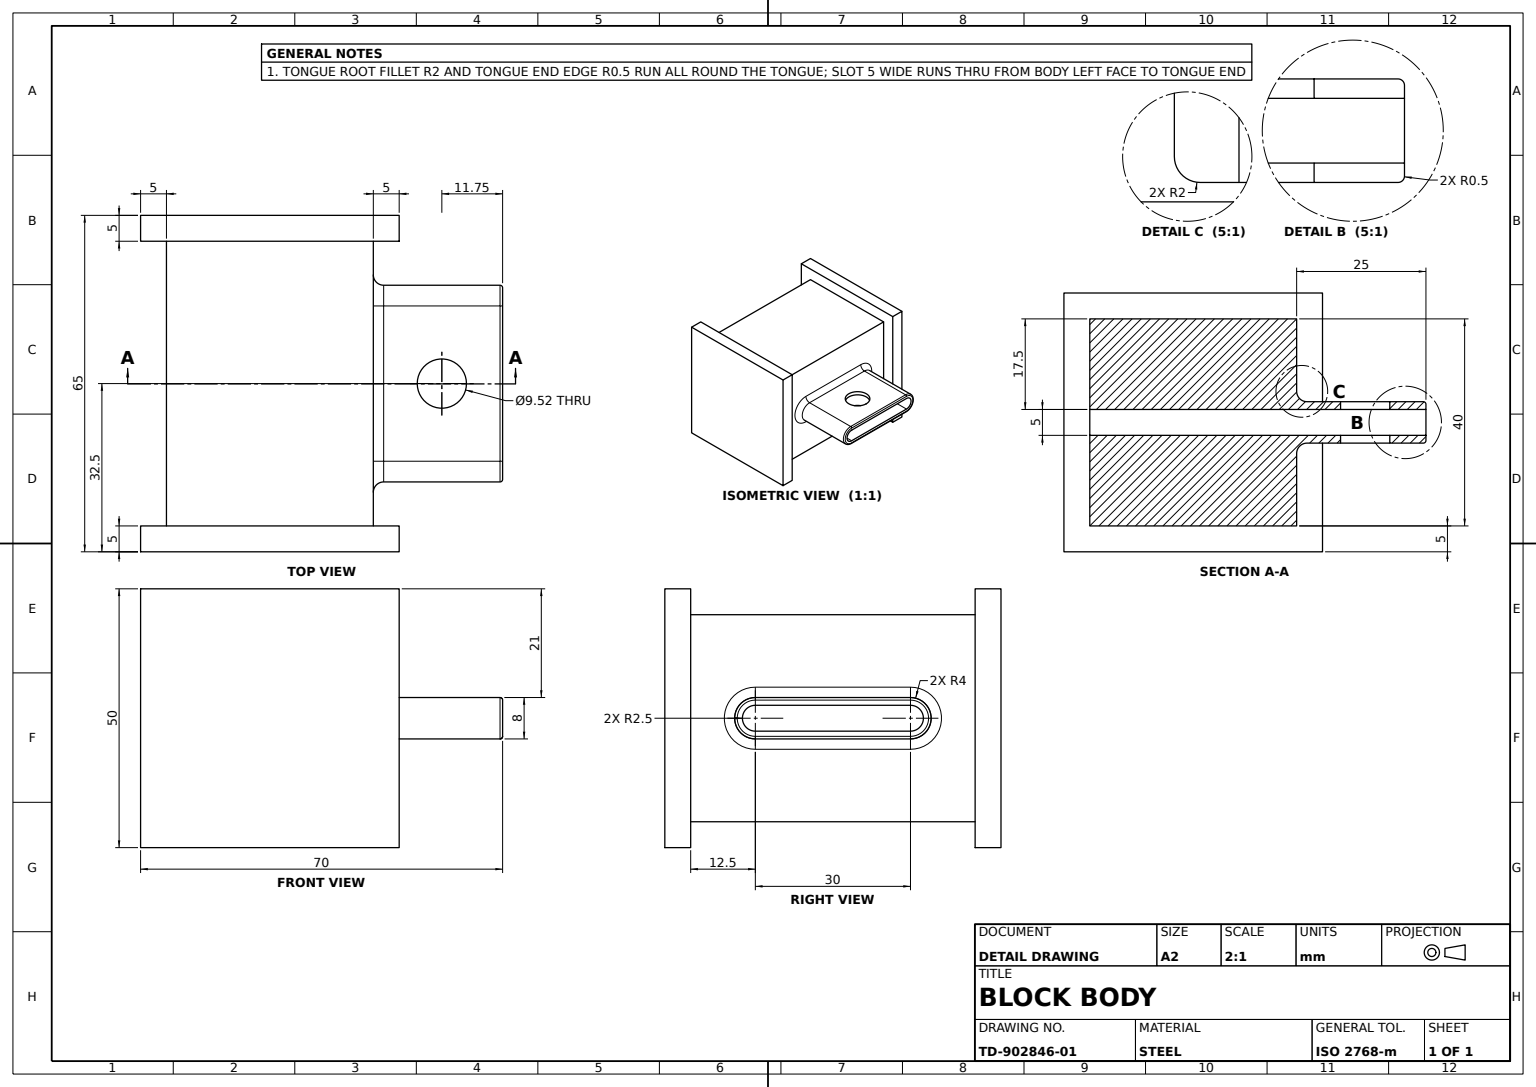
ISO-10303-21;
HEADER;
FILE_DESCRIPTION((''),'2;1');
FILE_NAME('','',(''),(''),'','','');
FILE_SCHEMA(('AUTOMOTIVE_DESIGN'));
ENDSEC;
DATA;
#1=APPLICATION_CONTEXT('');
#2=PRODUCT_CONTEXT('',#1,'mechanical');
#3=PRODUCT('','','',(#2));
#4=PRODUCT_DEFINITION_FORMATION('','',#3);
#5=PRODUCT_DEFINITION_CONTEXT('',#1,'design');
#6=PRODUCT_DEFINITION('','',#4,#5);
#7=PRODUCT_DEFINITION_SHAPE('','',#6);
#8=(LENGTH_UNIT()NAMED_UNIT(*)SI_UNIT(.MILLI.,.METRE.));
#9=(NAMED_UNIT(*)PLANE_ANGLE_UNIT()SI_UNIT($,.RADIAN.));
#10=(NAMED_UNIT(*)SI_UNIT($,.STERADIAN.)SOLID_ANGLE_UNIT());
#11=UNCERTAINTY_MEASURE_WITH_UNIT(LENGTH_MEASURE(1.E-05),#8,'distance_accuracy_value','');
#12=(GEOMETRIC_REPRESENTATION_CONTEXT(3)GLOBAL_UNCERTAINTY_ASSIGNED_CONTEXT((#11))GLOBAL_UNIT_ASSIGNED_CONTEXT((#8,#9,#10))REPRESENTATION_CONTEXT('',''));
#13=CARTESIAN_POINT('',(50.,0.,0.));
#14=VERTEX_POINT('',#13);
#15=CARTESIAN_POINT('',(50.,50.,0.));
#16=VERTEX_POINT('',#15);
#17=DIRECTION('',(0.,1.,0.));
#18=VECTOR('',#17,1000.);
#19=LINE('',#15,#18);
#20=EDGE_CURVE('',#14,#16,#19,.T.);
#21=ORIENTED_EDGE('',*,*,#20,.F.);
#22=CARTESIAN_POINT('',(0.,0.,0.));
#23=VERTEX_POINT('',#22);
#24=DIRECTION('',(1.,0.,0.));
#25=VECTOR('',#24,1000.);
#26=LINE('',#13,#25);
#27=EDGE_CURVE('',#23,#14,#26,.T.);
#28=ORIENTED_EDGE('',*,*,#27,.F.);
#29=CARTESIAN_POINT('',(0.,50.,0.));
#30=VERTEX_POINT('',#29);
#31=DIRECTION('',(0.,-1.,0.));
#32=VECTOR('',#31,1000.);
#33=LINE('',#22,#32);
#34=EDGE_CURVE('',#30,#23,#33,.T.);
#35=ORIENTED_EDGE('',*,*,#34,.F.);
#36=DIRECTION('',(-1.,0.,0.));
#37=VECTOR('',#36,1000.);
#38=LINE('',#29,#37);
#39=EDGE_CURVE('',#16,#30,#38,.T.);
#40=ORIENTED_EDGE('',*,*,#39,.F.);
#41=EDGE_LOOP('',(#21,#28,#35,#40));
#42=FACE_OUTER_BOUND('',#41,.T.);
#43=DIRECTION('',(0.,0.,-1.));
#44=AXIS2_PLACEMENT_3D('',#22,#43,#36);
#45=PLANE('',#44);
#46=ADVANCED_FACE('',(#42),#45,.T.);
#47=CARTESIAN_POINT('',(63.00949,29.,32.5));
#48=VERTEX_POINT('',#47);
#49=CARTESIAN_POINT('',(63.00949,27.5,32.5));
#50=VERTEX_POINT('',#49);
#51=CARTESIAN_POINT('',(63.00949,50.,32.5));
#52=LINE('',#51,#32);
#53=EDGE_CURVE('',#48,#50,#52,.T.);
#54=ORIENTED_EDGE('',*,*,#53,.F.);
#55=CARTESIAN_POINT('',(53.49051,29.,32.5));
#56=VERTEX_POINT('',#55);
#57=CARTESIAN_POINT('',(58.25,29.,32.5));
#58=AXIS2_PLACEMENT_3D('',#57,#17,#36);
#59=CIRCLE('',#58,4.75949);
#60=EDGE_CURVE('',#48,#56,#59,.T.);
#61=ORIENTED_EDGE('',*,*,#60,.T.);
#62=CARTESIAN_POINT('',(53.49051,27.5,32.5));
#63=VERTEX_POINT('',#62);
#64=CARTESIAN_POINT('',(53.49051,50.,32.5));
#65=LINE('',#64,#32);
#66=EDGE_CURVE('',#56,#63,#65,.T.);
#67=ORIENTED_EDGE('',*,*,#66,.T.);
#68=CARTESIAN_POINT('',(58.25,27.5,32.5));
#69=AXIS2_PLACEMENT_3D('',#68,#17,#36);
#70=CIRCLE('',#69,4.75949);
#71=EDGE_CURVE('',#50,#63,#70,.T.);
#72=ORIENTED_EDGE('',*,*,#71,.F.);
#73=EDGE_LOOP('',(#54,#61,#67,#72));
#74=FACE_OUTER_BOUND('',#73,.T.);
#75=CARTESIAN_POINT('',(58.25,50.,32.5));
#76=AXIS2_PLACEMENT_3D('',#75,#31,#24);
#77=CYLINDRICAL_SURFACE('',#76,4.75949);
#78=ADVANCED_FACE('',(#74),#77,.F.);
#79=CARTESIAN_POINT('',(5.,22.5,47.5));
#80=VERTEX_POINT('',#79);
#81=CARTESIAN_POINT('',(5.,22.5,17.5));
#82=VERTEX_POINT('',#81);
#83=CARTESIAN_POINT('',(5.,22.5,60.));
#84=VECTOR('',#43,1000.);
#85=LINE('',#83,#84);
#86=EDGE_CURVE('',#80,#82,#85,.T.);
#87=ORIENTED_EDGE('',*,*,#86,.T.);
#88=CARTESIAN_POINT('',(5.,27.5,17.5));
#89=VERTEX_POINT('',#88);
#90=CARTESIAN_POINT('',(5.,25.,17.5));
#91=AXIS2_PLACEMENT_3D('',#90,#24,#17);
#92=CIRCLE('',#91,2.5);
#93=EDGE_CURVE('',#82,#89,#92,.T.);
#94=ORIENTED_EDGE('',*,*,#93,.T.);
#95=CARTESIAN_POINT('',(5.,27.5,47.5));
#96=VERTEX_POINT('',#95);
#97=CARTESIAN_POINT('',(5.,27.5,60.));
#98=DIRECTION('',(0.,0.,1.));
#99=VECTOR('',#98,1000.);
#100=LINE('',#97,#99);
#101=EDGE_CURVE('',#89,#96,#100,.T.);
#102=ORIENTED_EDGE('',*,*,#101,.T.);
#103=CARTESIAN_POINT('',(5.,25.,47.5));
#104=AXIS2_PLACEMENT_3D('',#103,#24,#17);
#105=CIRCLE('',#104,2.5);
#106=EDGE_CURVE('',#96,#80,#105,.T.);
#107=ORIENTED_EDGE('',*,*,#106,.T.);
#108=EDGE_LOOP('',(#87,#94,#102,#107));
#109=FACE_BOUND('',#108,.T.);
#110=CARTESIAN_POINT('',(5.,45.,60.));
#111=VERTEX_POINT('',#110);
#112=CARTESIAN_POINT('',(5.,45.,5.));
#113=VERTEX_POINT('',#112);
#114=LINE('',#110,#84);
#115=EDGE_CURVE('',#111,#113,#114,.T.);
#116=ORIENTED_EDGE('',*,*,#115,.T.);
#117=CARTESIAN_POINT('',(5.,5.,5.));
#118=VERTEX_POINT('',#117);
#119=LINE('',#112,#32);
#120=EDGE_CURVE('',#113,#118,#119,.T.);
#121=ORIENTED_EDGE('',*,*,#120,.T.);
#122=CARTESIAN_POINT('',(5.,5.,60.));
#123=VERTEX_POINT('',#122);
#124=LINE('',#122,#84);
#125=EDGE_CURVE('',#123,#118,#124,.T.);
#126=ORIENTED_EDGE('',*,*,#125,.F.);
#127=LINE('',#110,#32);
#128=EDGE_CURVE('',#111,#123,#127,.T.);
#129=ORIENTED_EDGE('',*,*,#128,.F.);
#130=EDGE_LOOP('',(#116,#121,#126,#129));
#131=FACE_OUTER_BOUND('',#130,.T.);
#132=AXIS2_PLACEMENT_3D('',#110,#24,#17);
#133=PLANE('',#132);
#134=ADVANCED_FACE('',(#109,#131),#133,.F.);
#135=CARTESIAN_POINT('',(45.,5.,5.));
#136=VERTEX_POINT('',#135);
#137=LINE('',#117,#25);
#138=EDGE_CURVE('',#118,#136,#137,.T.);
#139=ORIENTED_EDGE('',*,*,#138,.T.);
#140=CARTESIAN_POINT('',(45.,5.,60.));
#141=VERTEX_POINT('',#140);
#142=LINE('',#140,#84);
#143=EDGE_CURVE('',#141,#136,#142,.T.);
#144=ORIENTED_EDGE('',*,*,#143,.F.);
#145=LINE('',#122,#25);
#146=EDGE_CURVE('',#123,#141,#145,.T.);
#147=ORIENTED_EDGE('',*,*,#146,.F.);
#148=ORIENTED_EDGE('',*,*,#125,.T.);
#149=EDGE_LOOP('',(#139,#144,#147,#148));
#150=FACE_OUTER_BOUND('',#149,.T.);
#151=AXIS2_PLACEMENT_3D('',#122,#17,#98);
#152=PLANE('',#151);
#153=ADVANCED_FACE('',(#150),#152,.F.);
#154=CARTESIAN_POINT('',(50.,50.,60.));
#155=VERTEX_POINT('',#154);
#156=CARTESIAN_POINT('',(0.,50.,60.));
#157=VERTEX_POINT('',#156);
#158=LINE('',#156,#37);
#159=EDGE_CURVE('',#155,#157,#158,.T.);
#160=ORIENTED_EDGE('',*,*,#159,.T.);
#161=CARTESIAN_POINT('',(0.,50.,65.));
#162=VERTEX_POINT('',#161);
#163=LINE('',#161,#84);
#164=EDGE_CURVE('',#162,#157,#163,.T.);
#165=ORIENTED_EDGE('',*,*,#164,.F.);
#166=CARTESIAN_POINT('',(50.,50.,65.));
#167=VERTEX_POINT('',#166);
#168=LINE('',#161,#37);
#169=EDGE_CURVE('',#167,#162,#168,.T.);
#170=ORIENTED_EDGE('',*,*,#169,.F.);
#171=LINE('',#166,#84);
#172=EDGE_CURVE('',#167,#155,#171,.T.);
#173=ORIENTED_EDGE('',*,*,#172,.T.);
#174=EDGE_LOOP('',(#160,#165,#170,#173));
#175=FACE_OUTER_BOUND('',#174,.T.);
#176=AXIS2_PLACEMENT_3D('',#161,#31,#43);
#177=PLANE('',#176);
#178=ADVANCED_FACE('',(#175),#177,.F.);
#179=CARTESIAN_POINT('',(47.,29.,17.5));
#180=VERTEX_POINT('',#179);
#181=CARTESIAN_POINT('',(47.,29.,47.5));
#182=VERTEX_POINT('',#181);
#183=LINE('',#181,#99);
#184=EDGE_CURVE('',#180,#182,#183,.T.);
#185=ORIENTED_EDGE('',*,*,#184,.F.);
#186=CARTESIAN_POINT('',(45.,31.,17.5));
#187=VERTEX_POINT('',#186);
#188=CARTESIAN_POINT('',(47.,31.,17.5));
#189=AXIS2_PLACEMENT_3D('',#188,#43,#36);
#190=CIRCLE('',#189,2.);
#191=EDGE_CURVE('',#180,#187,#190,.T.);
#192=ORIENTED_EDGE('',*,*,#191,.T.);
#193=CARTESIAN_POINT('',(45.,31.,47.5));
#194=VERTEX_POINT('',#193);
#195=CARTESIAN_POINT('',(45.,31.,60.));
#196=LINE('',#195,#84);
#197=EDGE_CURVE('',#194,#187,#196,.T.);
#198=ORIENTED_EDGE('',*,*,#197,.F.);
#199=CARTESIAN_POINT('',(47.,31.,47.5));
#200=AXIS2_PLACEMENT_3D('',#199,#43,#36);
#201=CIRCLE('',#200,2.);
#202=EDGE_CURVE('',#182,#194,#201,.T.);
#203=ORIENTED_EDGE('',*,*,#202,.F.);
#204=EDGE_LOOP('',(#185,#192,#198,#203));
#205=FACE_OUTER_BOUND('',#204,.T.);
#206=CARTESIAN_POINT('',(47.,31.,60.));
#207=AXIS2_PLACEMENT_3D('',#206,#43,#36);
#208=CYLINDRICAL_SURFACE('',#207,2.);
#209=ADVANCED_FACE('',(#205),#208,.F.);
#210=ORIENTED_EDGE('',*,*,#159,.F.);
#211=CARTESIAN_POINT('',(50.,0.,60.));
#212=VERTEX_POINT('',#211);
#213=LINE('',#154,#18);
#214=EDGE_CURVE('',#212,#155,#213,.T.);
#215=ORIENTED_EDGE('',*,*,#214,.F.);
#216=CARTESIAN_POINT('',(0.,0.,60.));
#217=VERTEX_POINT('',#216);
#218=LINE('',#211,#25);
#219=EDGE_CURVE('',#217,#212,#218,.T.);
#220=ORIENTED_EDGE('',*,*,#219,.F.);
#221=LINE('',#216,#32);
#222=EDGE_CURVE('',#157,#217,#221,.T.);
#223=ORIENTED_EDGE('',*,*,#222,.F.);
#224=EDGE_LOOP('',(#210,#215,#220,#223));
#225=FACE_OUTER_BOUND('',#224,.T.);
#226=ORIENTED_EDGE('',*,*,#128,.T.);
#227=ORIENTED_EDGE('',*,*,#146,.T.);
#228=CARTESIAN_POINT('',(45.,45.,60.));
#229=VERTEX_POINT('',#228);
#230=LINE('',#228,#18);
#231=EDGE_CURVE('',#141,#229,#230,.T.);
#232=ORIENTED_EDGE('',*,*,#231,.T.);
#233=LINE('',#110,#37);
#234=EDGE_CURVE('',#229,#111,#233,.T.);
#235=ORIENTED_EDGE('',*,*,#234,.T.);
#236=EDGE_LOOP('',(#226,#227,#232,#235));
#237=FACE_BOUND('',#236,.T.);
#238=AXIS2_PLACEMENT_3D('',#216,#43,#36);
#239=PLANE('',#238);
#240=ADVANCED_FACE('',(#225,#237),#239,.T.);
#241=CARTESIAN_POINT('',(45.,45.,5.));
#242=VERTEX_POINT('',#241);
#243=LINE('',#112,#37);
#244=EDGE_CURVE('',#242,#113,#243,.T.);
#245=ORIENTED_EDGE('',*,*,#244,.T.);
#246=ORIENTED_EDGE('',*,*,#115,.F.);
#247=ORIENTED_EDGE('',*,*,#234,.F.);
#248=LINE('',#228,#84);
#249=EDGE_CURVE('',#229,#242,#248,.T.);
#250=ORIENTED_EDGE('',*,*,#249,.T.);
#251=EDGE_LOOP('',(#245,#246,#247,#250));
#252=FACE_OUTER_BOUND('',#251,.T.);
#253=AXIS2_PLACEMENT_3D('',#110,#31,#43);
#254=PLANE('',#253);
#255=ADVANCED_FACE('',(#252),#254,.F.);
#256=CARTESIAN_POINT('',(69.5,21.,47.5));
#257=VERTEX_POINT('',#256);
#258=CARTESIAN_POINT('',(70.,21.5,47.5));
#259=VERTEX_POINT('',#258);
#260=CARTESIAN_POINT('',(69.5,21.5,47.5));
#261=AXIS2_PLACEMENT_3D('',#260,#98,#24);
#262=CIRCLE('',#261,0.5);
#263=EDGE_CURVE('',#257,#259,#262,.T.);
#264=ORIENTED_EDGE('',*,*,#263,.F.);
#265=CARTESIAN_POINT('',(69.5,21.,17.5));
#266=VERTEX_POINT('',#265);
#267=LINE('',#256,#99);
#268=EDGE_CURVE('',#266,#257,#267,.T.);
#269=ORIENTED_EDGE('',*,*,#268,.F.);
#270=CARTESIAN_POINT('',(70.,21.5,17.5));
#271=VERTEX_POINT('',#270);
#272=CARTESIAN_POINT('',(69.5,21.5,17.5));
#273=AXIS2_PLACEMENT_3D('',#272,#98,#24);
#274=CIRCLE('',#273,0.5);
#275=EDGE_CURVE('',#266,#271,#274,.T.);
#276=ORIENTED_EDGE('',*,*,#275,.T.);
#277=LINE('',#270,#84);
#278=EDGE_CURVE('',#259,#271,#277,.T.);
#279=ORIENTED_EDGE('',*,*,#278,.F.);
#280=EDGE_LOOP('',(#264,#269,#276,#279));
#281=FACE_OUTER_BOUND('',#280,.T.);
#282=CARTESIAN_POINT('',(69.5,21.5,0.));
#283=AXIS2_PLACEMENT_3D('',#282,#98,#24);
#284=CYLINDRICAL_SURFACE('',#283,0.5);
#285=ADVANCED_FACE('',(#281),#284,.T.);
#286=CARTESIAN_POINT('',(50.,0.,65.));
#287=VERTEX_POINT('',#286);
#288=LINE('',#166,#18);
#289=EDGE_CURVE('',#287,#167,#288,.T.);
#290=ORIENTED_EDGE('',*,*,#289,.F.);
#291=LINE('',#286,#84);
#292=EDGE_CURVE('',#287,#212,#291,.T.);
#293=ORIENTED_EDGE('',*,*,#292,.T.);
#294=ORIENTED_EDGE('',*,*,#214,.T.);
#295=ORIENTED_EDGE('',*,*,#172,.F.);
#296=EDGE_LOOP('',(#290,#293,#294,#295));
#297=FACE_OUTER_BOUND('',#296,.T.);
#298=AXIS2_PLACEMENT_3D('',#166,#36,#31);
#299=PLANE('',#298);
#300=ADVANCED_FACE('',(#297),#299,.F.);
#301=EDGE_CURVE('',#63,#50,#70,.T.);
#302=ORIENTED_EDGE('',*,*,#301,.T.);
#303=ORIENTED_EDGE('',*,*,#71,.T.);
#304=EDGE_LOOP('',(#302,#303));
#305=FACE_BOUND('',#304,.T.);
#306=CARTESIAN_POINT('',(70.,27.5,17.5));
#307=VERTEX_POINT('',#306);
#308=CARTESIAN_POINT('',(70.,27.5,47.5));
#309=VERTEX_POINT('',#308);
#310=LINE('',#306,#99);
#311=EDGE_CURVE('',#307,#309,#310,.T.);
#312=ORIENTED_EDGE('',*,*,#311,.T.);
#313=CARTESIAN_POINT('',(0.,27.5,47.5));
#314=LINE('',#313,#25);
#315=EDGE_CURVE('',#96,#309,#314,.T.);
#316=ORIENTED_EDGE('',*,*,#315,.F.);
#317=ORIENTED_EDGE('',*,*,#101,.F.);
#318=CARTESIAN_POINT('',(0.,27.5,17.5));
#319=LINE('',#318,#25);
#320=EDGE_CURVE('',#89,#307,#319,.T.);
#321=ORIENTED_EDGE('',*,*,#320,.T.);
#322=EDGE_LOOP('',(#312,#316,#317,#321));
#323=FACE_OUTER_BOUND('',#322,.T.);
#324=AXIS2_PLACEMENT_3D('',#318,#17,#36);
#325=PLANE('',#324);
#326=ADVANCED_FACE('',(#305,#323),#325,.F.);
#327=CARTESIAN_POINT('',(45.,19.,17.5));
#328=VERTEX_POINT('',#327);
#329=CARTESIAN_POINT('',(45.,25.,17.5));
#330=AXIS2_PLACEMENT_3D('',#329,#36,#31);
#331=CIRCLE('',#330,6.);
#332=EDGE_CURVE('',#187,#328,#331,.T.);
#333=ORIENTED_EDGE('',*,*,#332,.T.);
#334=CARTESIAN_POINT('',(45.,19.,47.5));
#335=VERTEX_POINT('',#334);
#336=LINE('',#334,#99);
#337=EDGE_CURVE('',#328,#335,#336,.T.);
#338=ORIENTED_EDGE('',*,*,#337,.T.);
#339=CARTESIAN_POINT('',(45.,25.,47.5));
#340=AXIS2_PLACEMENT_3D('',#339,#36,#31);
#341=CIRCLE('',#340,6.);
#342=EDGE_CURVE('',#335,#194,#341,.T.);
#343=ORIENTED_EDGE('',*,*,#342,.T.);
#344=ORIENTED_EDGE('',*,*,#197,.T.);
#345=EDGE_LOOP('',(#333,#338,#343,#344));
#346=FACE_BOUND('',#345,.T.);
#347=LINE('',#241,#18);
#348=EDGE_CURVE('',#136,#242,#347,.T.);
#349=ORIENTED_EDGE('',*,*,#348,.T.);
#350=ORIENTED_EDGE('',*,*,#249,.F.);
#351=ORIENTED_EDGE('',*,*,#231,.F.);
#352=ORIENTED_EDGE('',*,*,#143,.T.);
#353=EDGE_LOOP('',(#349,#350,#351,#352));
#354=FACE_OUTER_BOUND('',#353,.T.);
#355=AXIS2_PLACEMENT_3D('',#228,#36,#31);
#356=PLANE('',#355);
#357=ADVANCED_FACE('',(#346,#354),#356,.F.);
#358=ORIENTED_EDGE('',*,*,#138,.F.);
#359=ORIENTED_EDGE('',*,*,#120,.F.);
#360=ORIENTED_EDGE('',*,*,#244,.F.);
#361=ORIENTED_EDGE('',*,*,#348,.F.);
#362=EDGE_LOOP('',(#358,#359,#360,#361));
#363=FACE_BOUND('',#362,.T.);
#364=CARTESIAN_POINT('',(0.,0.,5.));
#365=VERTEX_POINT('',#364);
#366=CARTESIAN_POINT('',(50.,0.,5.));
#367=VERTEX_POINT('',#366);
#368=LINE('',#366,#25);
#369=EDGE_CURVE('',#365,#367,#368,.T.);
#370=ORIENTED_EDGE('',*,*,#369,.T.);
#371=CARTESIAN_POINT('',(50.,50.,5.));
#372=VERTEX_POINT('',#371);
#373=LINE('',#371,#18);
#374=EDGE_CURVE('',#367,#372,#373,.T.);
#375=ORIENTED_EDGE('',*,*,#374,.T.);
#376=CARTESIAN_POINT('',(0.,50.,5.));
#377=VERTEX_POINT('',#376);
#378=LINE('',#376,#37);
#379=EDGE_CURVE('',#372,#377,#378,.T.);
#380=ORIENTED_EDGE('',*,*,#379,.T.);
#381=LINE('',#364,#32);
#382=EDGE_CURVE('',#377,#365,#381,.T.);
#383=ORIENTED_EDGE('',*,*,#382,.T.);
#384=EDGE_LOOP('',(#370,#375,#380,#383));
#385=FACE_OUTER_BOUND('',#384,.T.);
#386=AXIS2_PLACEMENT_3D('',#364,#43,#36);
#387=PLANE('',#386);
#388=ADVANCED_FACE('',(#363,#385),#387,.F.);
#389=LINE('',#376,#84);
#390=EDGE_CURVE('',#377,#30,#389,.T.);
#391=ORIENTED_EDGE('',*,*,#390,.F.);
#392=ORIENTED_EDGE('',*,*,#379,.F.);
#393=LINE('',#371,#84);
#394=EDGE_CURVE('',#372,#16,#393,.T.);
#395=ORIENTED_EDGE('',*,*,#394,.T.);
#396=ORIENTED_EDGE('',*,*,#39,.T.);
#397=EDGE_LOOP('',(#391,#392,#395,#396));
#398=FACE_OUTER_BOUND('',#397,.T.);
#399=AXIS2_PLACEMENT_3D('',#376,#31,#43);
#400=PLANE('',#399);
#401=ADVANCED_FACE('',(#398),#400,.F.);
#402=CARTESIAN_POINT('',(53.49051,22.5,32.5));
#403=VERTEX_POINT('',#402);
#404=CARTESIAN_POINT('',(63.00949,22.5,32.5));
#405=VERTEX_POINT('',#404);
#406=CARTESIAN_POINT('',(58.25,22.5,32.5));
#407=AXIS2_PLACEMENT_3D('',#406,#31,#24);
#408=CIRCLE('',#407,4.75949);
#409=EDGE_CURVE('',#403,#405,#408,.T.);
#410=ORIENTED_EDGE('',*,*,#409,.F.);
#411=CARTESIAN_POINT('',(53.49051,21.,32.5));
#412=VERTEX_POINT('',#411);
#413=EDGE_CURVE('',#403,#412,#65,.T.);
#414=ORIENTED_EDGE('',*,*,#413,.T.);
#415=CARTESIAN_POINT('',(63.00949,21.,32.5));
#416=VERTEX_POINT('',#415);
#417=CARTESIAN_POINT('',(58.25,21.,32.5));
#418=AXIS2_PLACEMENT_3D('',#417,#31,#24);
#419=CIRCLE('',#418,4.75949);
#420=EDGE_CURVE('',#412,#416,#419,.T.);
#421=ORIENTED_EDGE('',*,*,#420,.T.);
#422=EDGE_CURVE('',#405,#416,#52,.T.);
#423=ORIENTED_EDGE('',*,*,#422,.F.);
#424=EDGE_LOOP('',(#410,#414,#421,#423));
#425=FACE_OUTER_BOUND('',#424,.T.);
#426=ADVANCED_FACE('',(#425),#77,.F.);
#427=CARTESIAN_POINT('',(47.,21.,17.5));
#428=VERTEX_POINT('',#427);
#429=CARTESIAN_POINT('',(47.,19.,17.5));
#430=AXIS2_PLACEMENT_3D('',#429,#43,#36);
#431=CIRCLE('',#430,2.);
#432=EDGE_CURVE('',#328,#428,#431,.T.);
#433=ORIENTED_EDGE('',*,*,#432,.F.);
#434=ORIENTED_EDGE('',*,*,#332,.F.);
#435=ORIENTED_EDGE('',*,*,#191,.F.);
#436=CARTESIAN_POINT('',(47.,25.,17.5));
#437=AXIS2_PLACEMENT_3D('',#436,#24,#31);
#438=CIRCLE('',#437,4.);
#439=EDGE_CURVE('',#428,#180,#438,.T.);
#440=ORIENTED_EDGE('',*,*,#439,.F.);
#441=EDGE_LOOP('',(#433,#434,#435,#440));
#442=FACE_OUTER_BOUND('',#441,.T.);
#443=AXIS2_PLACEMENT_3D('',#436,#36,#31);
#444=TOROIDAL_SURFACE('',#443,6.,2.);
#445=ADVANCED_FACE('',(#442),#444,.F.);
#446=ORIENTED_EDGE('',*,*,#409,.T.);
#447=EDGE_CURVE('',#405,#403,#408,.T.);
#448=ORIENTED_EDGE('',*,*,#447,.T.);
#449=EDGE_LOOP('',(#446,#448));
#450=FACE_BOUND('',#449,.T.);
#451=CARTESIAN_POINT('',(70.,22.5,47.5));
#452=VERTEX_POINT('',#451);
#453=CARTESIAN_POINT('',(0.,22.5,47.5));
#454=LINE('',#453,#25);
#455=EDGE_CURVE('',#80,#452,#454,.T.);
#456=ORIENTED_EDGE('',*,*,#455,.T.);
#457=CARTESIAN_POINT('',(70.,22.5,17.5));
#458=VERTEX_POINT('',#457);
#459=LINE('',#451,#84);
#460=EDGE_CURVE('',#452,#458,#459,.T.);
#461=ORIENTED_EDGE('',*,*,#460,.T.);
#462=CARTESIAN_POINT('',(0.,22.5,17.5));
#463=LINE('',#462,#25);
#464=EDGE_CURVE('',#82,#458,#463,.T.);
#465=ORIENTED_EDGE('',*,*,#464,.F.);
#466=ORIENTED_EDGE('',*,*,#86,.F.);
#467=EDGE_LOOP('',(#456,#461,#465,#466));
#468=FACE_OUTER_BOUND('',#467,.T.);
#469=AXIS2_PLACEMENT_3D('',#453,#31,#24);
#470=PLANE('',#469);
#471=ADVANCED_FACE('',(#450,#468),#470,.F.);
#472=ORIENTED_EDGE('',*,*,#93,.F.);
#473=ORIENTED_EDGE('',*,*,#464,.T.);
#474=CARTESIAN_POINT('',(70.,25.,17.5));
#475=AXIS2_PLACEMENT_3D('',#474,#24,#17);
#476=CIRCLE('',#475,2.5);
#477=EDGE_CURVE('',#458,#307,#476,.T.);
#478=ORIENTED_EDGE('',*,*,#477,.T.);
#479=ORIENTED_EDGE('',*,*,#320,.F.);
#480=EDGE_LOOP('',(#472,#473,#478,#479));
#481=FACE_OUTER_BOUND('',#480,.T.);
#482=CARTESIAN_POINT('',(0.,25.,17.5));
#483=AXIS2_PLACEMENT_3D('',#482,#24,#17);
#484=CYLINDRICAL_SURFACE('',#483,2.5);
#485=ADVANCED_FACE('',(#481),#484,.F.);
#486=ORIENTED_EDGE('',*,*,#342,.F.);
#487=CARTESIAN_POINT('',(47.,21.,47.5));
#488=VERTEX_POINT('',#487);
#489=CARTESIAN_POINT('',(47.,19.,47.5));
#490=AXIS2_PLACEMENT_3D('',#489,#43,#36);
#491=CIRCLE('',#490,2.);
#492=EDGE_CURVE('',#335,#488,#491,.T.);
#493=ORIENTED_EDGE('',*,*,#492,.T.);
#494=CARTESIAN_POINT('',(47.,25.,47.5));
#495=AXIS2_PLACEMENT_3D('',#494,#24,#31);
#496=CIRCLE('',#495,4.);
#497=EDGE_CURVE('',#182,#488,#496,.T.);
#498=ORIENTED_EDGE('',*,*,#497,.F.);
#499=ORIENTED_EDGE('',*,*,#202,.T.);
#500=EDGE_LOOP('',(#486,#493,#498,#499));
#501=FACE_OUTER_BOUND('',#500,.T.);
#502=AXIS2_PLACEMENT_3D('',#494,#36,#31);
#503=TOROIDAL_SURFACE('',#502,6.,2.);
#504=ADVANCED_FACE('',(#501),#503,.F.);
#505=ORIENTED_EDGE('',*,*,#439,.T.);
#506=CARTESIAN_POINT('',(69.5,29.,17.5));
#507=VERTEX_POINT('',#506);
#508=CARTESIAN_POINT('',(70.,29.,17.5));
#509=LINE('',#508,#37);
#510=EDGE_CURVE('',#507,#180,#509,.T.);
#511=ORIENTED_EDGE('',*,*,#510,.F.);
#512=CARTESIAN_POINT('',(69.5,25.,17.5));
#513=AXIS2_PLACEMENT_3D('',#512,#36,#17);
#514=CIRCLE('',#513,4.);
#515=EDGE_CURVE('',#507,#266,#514,.T.);
#516=ORIENTED_EDGE('',*,*,#515,.T.);
#517=CARTESIAN_POINT('',(70.,21.,17.5));
#518=LINE('',#517,#37);
#519=EDGE_CURVE('',#266,#428,#518,.T.);
#520=ORIENTED_EDGE('',*,*,#519,.T.);
#521=EDGE_LOOP('',(#505,#511,#516,#520));
#522=FACE_OUTER_BOUND('',#521,.T.);
#523=AXIS2_PLACEMENT_3D('',#474,#36,#31);
#524=CYLINDRICAL_SURFACE('',#523,4.);
#525=ADVANCED_FACE('',(#522),#524,.T.);
#526=ORIENTED_EDGE('',*,*,#374,.F.);
#527=LINE('',#366,#84);
#528=EDGE_CURVE('',#367,#14,#527,.T.);
#529=ORIENTED_EDGE('',*,*,#528,.T.);
#530=ORIENTED_EDGE('',*,*,#20,.T.);
#531=ORIENTED_EDGE('',*,*,#394,.F.);
#532=EDGE_LOOP('',(#526,#529,#530,#531));
#533=FACE_OUTER_BOUND('',#532,.T.);
#534=AXIS2_PLACEMENT_3D('',#371,#36,#31);
#535=PLANE('',#534);
#536=ADVANCED_FACE('',(#533),#535,.F.);
#537=CARTESIAN_POINT('',(0.,0.,65.));
#538=VERTEX_POINT('',#537);
#539=LINE('',#537,#32);
#540=EDGE_CURVE('',#162,#538,#539,.T.);
#541=ORIENTED_EDGE('',*,*,#540,.F.);
#542=ORIENTED_EDGE('',*,*,#164,.T.);
#543=ORIENTED_EDGE('',*,*,#222,.T.);
#544=LINE('',#537,#84);
#545=EDGE_CURVE('',#538,#217,#544,.T.);
#546=ORIENTED_EDGE('',*,*,#545,.F.);
#547=EDGE_LOOP('',(#541,#542,#543,#546));
#548=FACE_OUTER_BOUND('',#547,.T.);
#549=AXIS2_PLACEMENT_3D('',#537,#24,#43);
#550=PLANE('',#549);
#551=ADVANCED_FACE('',(#548),#550,.F.);
#552=CARTESIAN_POINT('',(70.,28.5,17.5));
#553=VERTEX_POINT('',#552);
#554=CIRCLE('',#475,3.5);
#555=EDGE_CURVE('',#271,#553,#554,.T.);
#556=ORIENTED_EDGE('',*,*,#555,.F.);
#557=ORIENTED_EDGE('',*,*,#275,.F.);
#558=ORIENTED_EDGE('',*,*,#515,.F.);
#559=CARTESIAN_POINT('',(69.5,28.5,17.5));
#560=AXIS2_PLACEMENT_3D('',#559,#98,#24);
#561=CIRCLE('',#560,0.5);
#562=EDGE_CURVE('',#553,#507,#561,.T.);
#563=ORIENTED_EDGE('',*,*,#562,.F.);
#564=EDGE_LOOP('',(#556,#557,#558,#563));
#565=FACE_OUTER_BOUND('',#564,.T.);
#566=AXIS2_PLACEMENT_3D('',#512,#24,#17);
#567=TOROIDAL_SURFACE('',#566,3.5,0.5);
#568=ADVANCED_FACE('',(#565),#567,.T.);
#569=CARTESIAN_POINT('',(70.,25.,47.5));
#570=AXIS2_PLACEMENT_3D('',#569,#24,#17);
#571=CIRCLE('',#570,2.5);
#572=EDGE_CURVE('',#309,#452,#571,.T.);
#573=ORIENTED_EDGE('',*,*,#572,.F.);
#574=ORIENTED_EDGE('',*,*,#311,.F.);
#575=ORIENTED_EDGE('',*,*,#477,.F.);
#576=ORIENTED_EDGE('',*,*,#460,.F.);
#577=EDGE_LOOP('',(#573,#574,#575,#576));
#578=FACE_BOUND('',#577,.T.);
#579=ORIENTED_EDGE('',*,*,#278,.T.);
#580=ORIENTED_EDGE('',*,*,#555,.T.);
#581=CARTESIAN_POINT('',(70.,28.5,47.5));
#582=VERTEX_POINT('',#581);
#583=CARTESIAN_POINT('',(70.,28.5,0.));
#584=LINE('',#583,#99);
#585=EDGE_CURVE('',#553,#582,#584,.T.);
#586=ORIENTED_EDGE('',*,*,#585,.T.);
#587=CIRCLE('',#570,3.5);
#588=EDGE_CURVE('',#582,#259,#587,.T.);
#589=ORIENTED_EDGE('',*,*,#588,.T.);
#590=EDGE_LOOP('',(#579,#580,#586,#589));
#591=FACE_OUTER_BOUND('',#590,.T.);
#592=CARTESIAN_POINT('',(70.,0.,0.));
#593=AXIS2_PLACEMENT_3D('',#592,#24,#17);
#594=PLANE('',#593);
#595=ADVANCED_FACE('',(#578,#591),#594,.T.);
#596=ORIENTED_EDGE('',*,*,#497,.T.);
#597=CARTESIAN_POINT('',(70.,21.,47.5));
#598=LINE('',#597,#37);
#599=EDGE_CURVE('',#257,#488,#598,.T.);
#600=ORIENTED_EDGE('',*,*,#599,.F.);
#601=CARTESIAN_POINT('',(69.5,29.,47.5));
#602=VERTEX_POINT('',#601);
#603=CARTESIAN_POINT('',(69.5,25.,47.5));
#604=AXIS2_PLACEMENT_3D('',#603,#36,#17);
#605=CIRCLE('',#604,4.);
#606=EDGE_CURVE('',#257,#602,#605,.T.);
#607=ORIENTED_EDGE('',*,*,#606,.T.);
#608=CARTESIAN_POINT('',(70.,29.,47.5));
#609=LINE('',#608,#37);
#610=EDGE_CURVE('',#602,#182,#609,.T.);
#611=ORIENTED_EDGE('',*,*,#610,.T.);
#612=EDGE_LOOP('',(#596,#600,#607,#611));
#613=FACE_OUTER_BOUND('',#612,.T.);
#614=AXIS2_PLACEMENT_3D('',#569,#36,#31);
#615=CYLINDRICAL_SURFACE('',#614,4.);
#616=ADVANCED_FACE('',(#613),#615,.T.);
#617=ORIENTED_EDGE('',*,*,#585,.F.);
#618=ORIENTED_EDGE('',*,*,#562,.T.);
#619=LINE('',#601,#84);
#620=EDGE_CURVE('',#602,#507,#619,.T.);
#621=ORIENTED_EDGE('',*,*,#620,.F.);
#622=CARTESIAN_POINT('',(69.5,28.5,47.5));
#623=AXIS2_PLACEMENT_3D('',#622,#98,#24);
#624=CIRCLE('',#623,0.5);
#625=EDGE_CURVE('',#582,#602,#624,.T.);
#626=ORIENTED_EDGE('',*,*,#625,.F.);
#627=EDGE_LOOP('',(#617,#618,#621,#626));
#628=FACE_OUTER_BOUND('',#627,.T.);
#629=AXIS2_PLACEMENT_3D('',#622,#43,#36);
#630=CYLINDRICAL_SURFACE('',#629,0.5);
#631=ADVANCED_FACE('',(#628),#630,.T.);
#632=ORIENTED_EDGE('',*,*,#572,.T.);
#633=ORIENTED_EDGE('',*,*,#455,.F.);
#634=ORIENTED_EDGE('',*,*,#106,.F.);
#635=ORIENTED_EDGE('',*,*,#315,.T.);
#636=EDGE_LOOP('',(#632,#633,#634,#635));
#637=FACE_OUTER_BOUND('',#636,.T.);
#638=CARTESIAN_POINT('',(0.,25.,47.5));
#639=AXIS2_PLACEMENT_3D('',#638,#24,#17);
#640=CYLINDRICAL_SURFACE('',#639,2.5);
#641=ADVANCED_FACE('',(#637),#640,.F.);
#642=ORIENTED_EDGE('',*,*,#588,.F.);
#643=ORIENTED_EDGE('',*,*,#625,.T.);
#644=ORIENTED_EDGE('',*,*,#606,.F.);
#645=ORIENTED_EDGE('',*,*,#263,.T.);
#646=EDGE_LOOP('',(#642,#643,#644,#645));
#647=FACE_OUTER_BOUND('',#646,.T.);
#648=AXIS2_PLACEMENT_3D('',#603,#24,#17);
#649=TOROIDAL_SURFACE('',#648,3.5,0.5);
#650=ADVANCED_FACE('',(#647),#649,.T.);
#651=ORIENTED_EDGE('',*,*,#27,.T.);
#652=ORIENTED_EDGE('',*,*,#528,.F.);
#653=ORIENTED_EDGE('',*,*,#369,.F.);
#654=LINE('',#364,#84);
#655=EDGE_CURVE('',#365,#23,#654,.T.);
#656=ORIENTED_EDGE('',*,*,#655,.T.);
#657=EDGE_LOOP('',(#651,#652,#653,#656));
#658=FACE_OUTER_BOUND('',#657,.T.);
#659=AXIS2_PLACEMENT_3D('',#366,#17,#36);
#660=PLANE('',#659);
#661=ADVANCED_FACE('',(#658),#660,.F.);
#662=ORIENTED_EDGE('',*,*,#492,.F.);
#663=ORIENTED_EDGE('',*,*,#337,.F.);
#664=ORIENTED_EDGE('',*,*,#432,.T.);
#665=LINE('',#427,#84);
#666=EDGE_CURVE('',#488,#428,#665,.T.);
#667=ORIENTED_EDGE('',*,*,#666,.F.);
#668=EDGE_LOOP('',(#662,#663,#664,#667));
#669=FACE_OUTER_BOUND('',#668,.T.);
#670=CARTESIAN_POINT('',(47.,19.,0.));
#671=AXIS2_PLACEMENT_3D('',#670,#98,#24);
#672=CYLINDRICAL_SURFACE('',#671,2.);
#673=ADVANCED_FACE('',(#669),#672,.F.);
#674=ORIENTED_EDGE('',*,*,#422,.T.);
#675=EDGE_CURVE('',#416,#412,#419,.T.);
#676=ORIENTED_EDGE('',*,*,#675,.T.);
#677=ORIENTED_EDGE('',*,*,#413,.F.);
#678=ORIENTED_EDGE('',*,*,#447,.F.);
#679=EDGE_LOOP('',(#674,#676,#677,#678));
#680=FACE_OUTER_BOUND('',#679,.T.);
#681=ADVANCED_FACE('',(#680),#77,.F.);
#682=LINE('',#286,#25);
#683=EDGE_CURVE('',#538,#287,#682,.T.);
#684=ORIENTED_EDGE('',*,*,#683,.T.);
#685=ORIENTED_EDGE('',*,*,#289,.T.);
#686=ORIENTED_EDGE('',*,*,#169,.T.);
#687=ORIENTED_EDGE('',*,*,#540,.T.);
#688=EDGE_LOOP('',(#684,#685,#686,#687));
#689=FACE_OUTER_BOUND('',#688,.T.);
#690=AXIS2_PLACEMENT_3D('',#537,#43,#36);
#691=PLANE('',#690);
#692=ADVANCED_FACE('',(#689),#691,.F.);
#693=ORIENTED_EDGE('',*,*,#219,.T.);
#694=ORIENTED_EDGE('',*,*,#292,.F.);
#695=ORIENTED_EDGE('',*,*,#683,.F.);
#696=ORIENTED_EDGE('',*,*,#545,.T.);
#697=EDGE_LOOP('',(#693,#694,#695,#696));
#698=FACE_OUTER_BOUND('',#697,.T.);
#699=AXIS2_PLACEMENT_3D('',#286,#17,#36);
#700=PLANE('',#699);
#701=ADVANCED_FACE('',(#698),#700,.F.);
#702=EDGE_CURVE('',#56,#48,#59,.T.);
#703=ORIENTED_EDGE('',*,*,#702,.F.);
#704=ORIENTED_EDGE('',*,*,#60,.F.);
#705=EDGE_LOOP('',(#703,#704));
#706=FACE_BOUND('',#705,.T.);
#707=ORIENTED_EDGE('',*,*,#184,.T.);
#708=ORIENTED_EDGE('',*,*,#610,.F.);
#709=ORIENTED_EDGE('',*,*,#620,.T.);
#710=ORIENTED_EDGE('',*,*,#510,.T.);
#711=EDGE_LOOP('',(#707,#708,#709,#710));
#712=FACE_OUTER_BOUND('',#711,.T.);
#713=AXIS2_PLACEMENT_3D('',#608,#17,#36);
#714=PLANE('',#713);
#715=ADVANCED_FACE('',(#706,#712),#714,.T.);
#716=ORIENTED_EDGE('',*,*,#675,.F.);
#717=ORIENTED_EDGE('',*,*,#420,.F.);
#718=EDGE_LOOP('',(#716,#717));
#719=FACE_BOUND('',#718,.T.);
#720=ORIENTED_EDGE('',*,*,#666,.T.);
#721=ORIENTED_EDGE('',*,*,#519,.F.);
#722=ORIENTED_EDGE('',*,*,#268,.T.);
#723=ORIENTED_EDGE('',*,*,#599,.T.);
#724=EDGE_LOOP('',(#720,#721,#722,#723));
#725=FACE_OUTER_BOUND('',#724,.T.);
#726=CARTESIAN_POINT('',(70.,21.,0.));
#727=AXIS2_PLACEMENT_3D('',#726,#17,#36);
#728=PLANE('',#727);
#729=ADVANCED_FACE('',(#719,#725),#728,.F.);
#730=ORIENTED_EDGE('',*,*,#702,.T.);
#731=ORIENTED_EDGE('',*,*,#53,.T.);
#732=ORIENTED_EDGE('',*,*,#301,.F.);
#733=ORIENTED_EDGE('',*,*,#66,.F.);
#734=EDGE_LOOP('',(#730,#731,#732,#733));
#735=FACE_OUTER_BOUND('',#734,.T.);
#736=ADVANCED_FACE('',(#735),#77,.F.);
#737=ORIENTED_EDGE('',*,*,#655,.F.);
#738=ORIENTED_EDGE('',*,*,#382,.F.);
#739=ORIENTED_EDGE('',*,*,#390,.T.);
#740=ORIENTED_EDGE('',*,*,#34,.T.);
#741=EDGE_LOOP('',(#737,#738,#739,#740));
#742=FACE_OUTER_BOUND('',#741,.T.);
#743=AXIS2_PLACEMENT_3D('',#364,#24,#43);
#744=PLANE('',#743);
#745=ADVANCED_FACE('',(#742),#744,.F.);
#746=CLOSED_SHELL('',(#46,#78,#134,#153,#178,#209,#240,#255,#285,#300,#326,#357,#388,#401,#426,#445,#471,#485,#504,#525,#536,#551,#568,#595,#616,#631,#641,#650,#661,#673,#681,#692,#701,#715,#729,#736,#745));
#747=MANIFOLD_SOLID_BREP('',#746);
#748=ADVANCED_BREP_SHAPE_REPRESENTATION('',(#747),#12);
#749=SHAPE_DEFINITION_REPRESENTATION(#7,#748);
ENDSEC;
END-ISO-10303-21;
